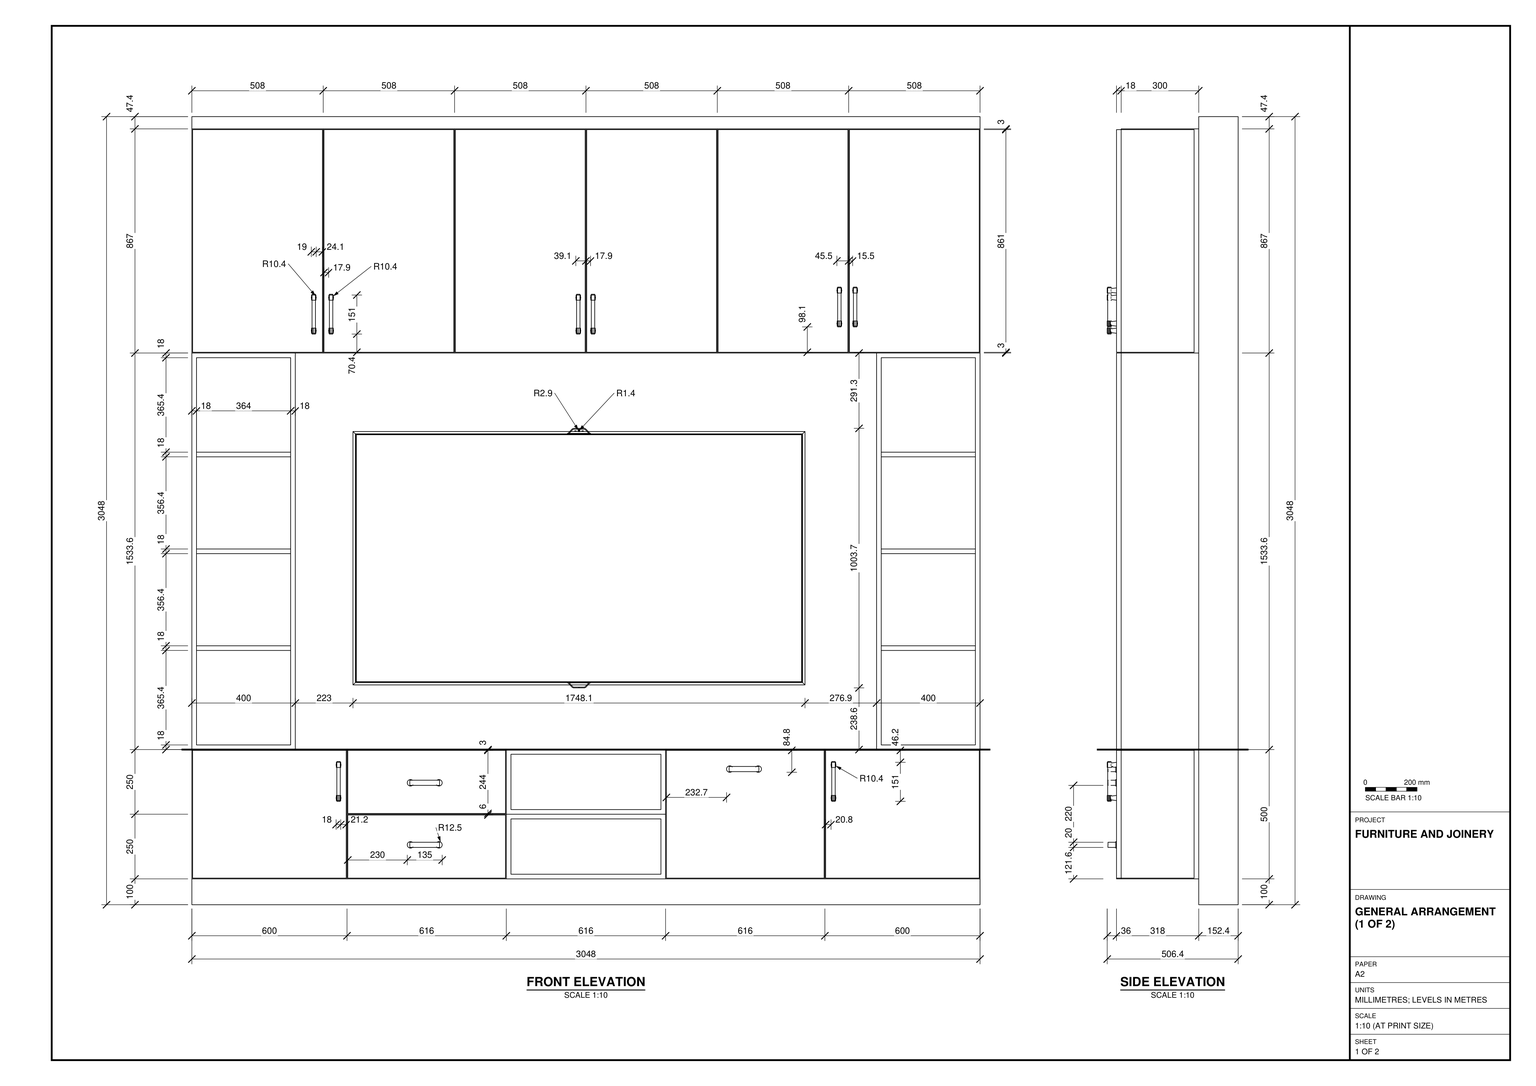
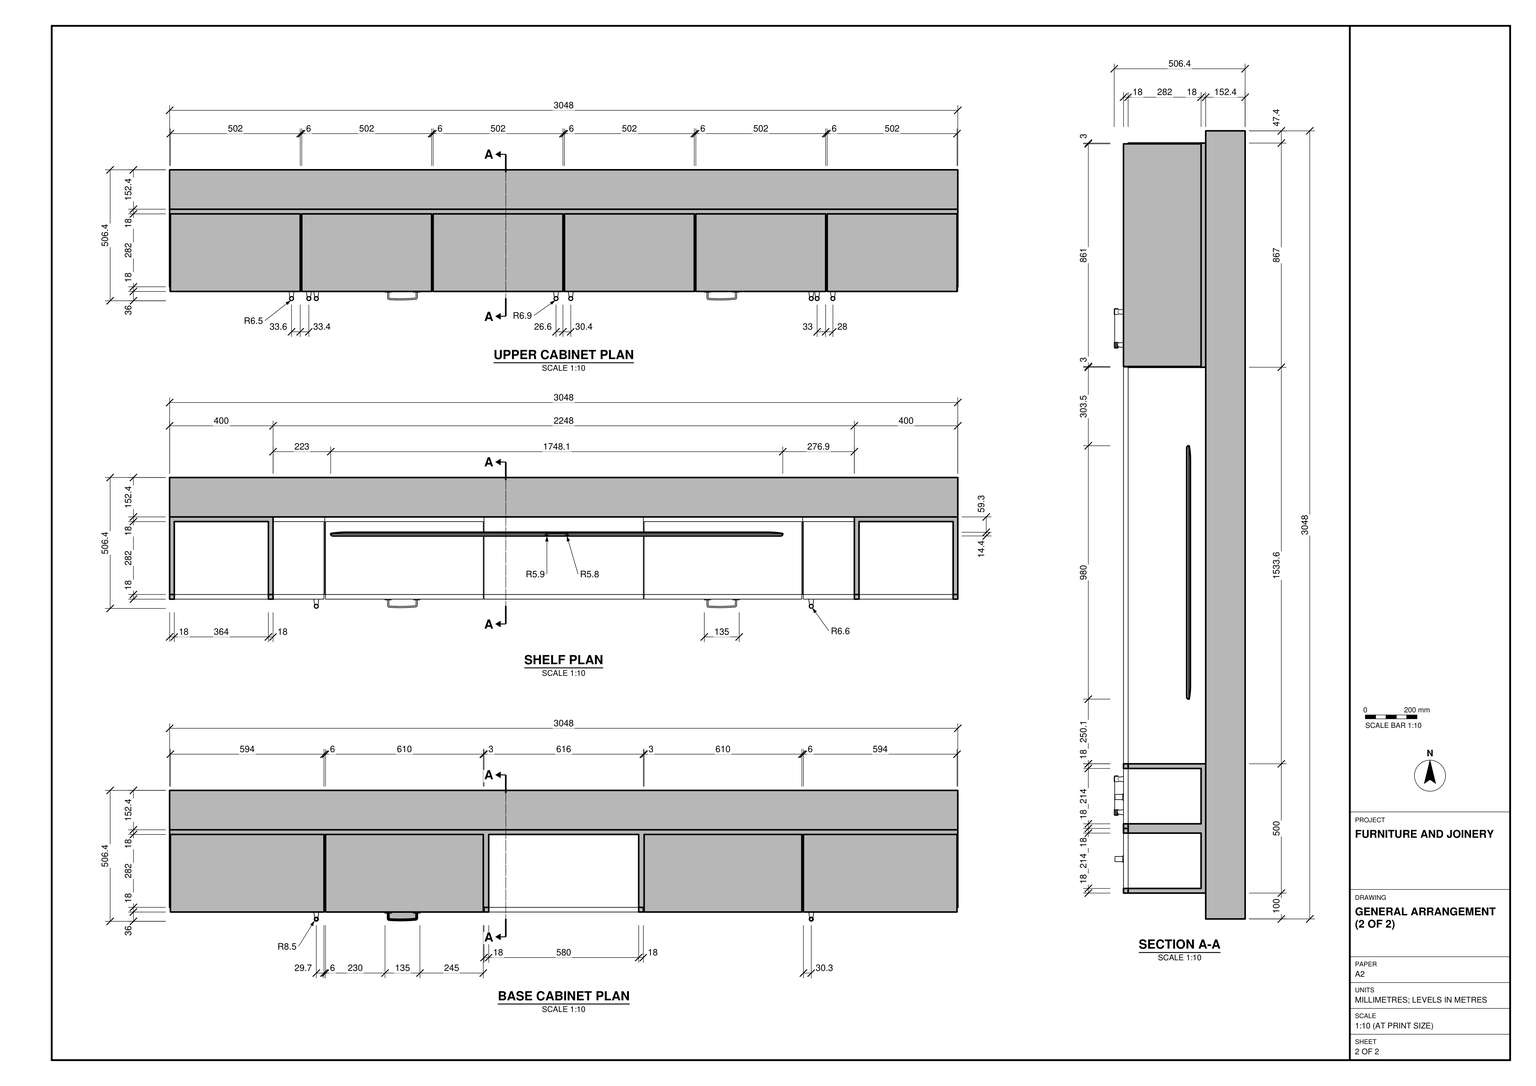
Build the television wall unit in SketchUp from task_files/diagram_01.pdf. Work in millimetres and use 0 mm as the floor datum. The complete assembly is 3048 mm wide, 506.4 mm deep and 3048 mm high. Use the front elevation to lay out the cabinet fronts and the plans and section to set their depths relative to the 152.4 mm thick backing wall.

Set the base cabinets 100 mm above the floor. Across the base, model an end cupboard, two stacked drawers, two stacked open compartments, a single full-height front and the other end cupboard, in that order. Above the base, build a 400 mm wide open shelving tower at each end. Mount the television against the backing between the towers, leaving the slightly larger clearance on its right shown in the shelf plan. Span the full width above the towers with six upper cabinet doors. Match the panel thicknesses, gaps between fronts and handle positions to the drawings.

Keep the backing wall, cabinet assemblies, shelving towers and television as separate groups or components, and use components for repeated parts such as shelves and handles. Decor and loose items, including the television, may use any suitable library component. Save one SketchUp model as output_files/television_wall_unit_with_cabinets_and_open_shelving.skp.

# SketchUp Ruby script. Lengths in millimetres.
U = 1.mm
M = Sketchup.active_model
def pt(a) = Geom::Point3d.new(a.map { |v| v * U })
def face(e, loops, mat)
  f = e.add_face(loops[0].map { |a| pt(a) })
  loops[1..].each { |l| e.add_face(l.map { |a| pt(a) }).erase! }
  f.material = f.back_material = mat if mat
  f
end
# faces: each face lists its corners as indices into pts; further lists are holes
def faces(e, pts, list, mat = nil) = list.each { |f| face(e, (f[0].is_a?(Array) ? f : [f]).map { |l| l.map { |i| pts[i] } }, mat) }
# xy, xz, yz: faces in a plane at the given z, y or x. An outline is a flat list of corners, or four numbers for a rectangle; further outlines are holes
def ring(l) = l.size == 4 ? [[l[0], l[1]], [l[2], l[1]], [l[2], l[3]], [l[0], l[3]]] : l.each_slice(2).to_a
def flat(e, list, mat, &to3) = list.each { |f| face(e, (f[0].is_a?(Array) ? f : [f]).map { |l| ring(l).map { |u, v| to3.(u, v) } }, mat) }
def xy(e, z, list, mat = nil) = flat(e, list, mat) { |x, y| [x, y, z] }
def xz(e, y, list, mat = nil) = flat(e, list, mat) { |x, z| [x, y, z] }
def yz(e, x, list, mat = nil) = flat(e, list, mat) { |y, z| [x, y, z] }
def lines(e, pts, list) = list.each { |a, b| e.add_line(pt(pts[a]), pt(pts[b])) }
# prism: a flat outline (further loops are holes) pulled along v
def prism(e, loops, v, mat = nil)
  f = face(e, loops, mat); d = Geom::Vector3d.new(v.map { |x| x * U })
  f.pushpull(f.normal.samedirection?(d) ? d.length : -d.length)
end
def box(e, o, s, mat = nil) = prism(e, [[o, [o[0] + s[0], o[1], o[2]], [o[0] + s[0], o[1] + s[1], o[2]], [o[0], o[1] + s[1], o[2]]]], [0, 0, s[2]], mat)
def at(x, y, z, deg = 0) = Geom::Transformation.translation(pt([x, y, z])) * Geom::Transformation.rotation(ORIGIN, Z_AXIS, deg.degrees)
def axes(o, x, y, z) = Geom::Transformation.new([*x, 0, *y, 0, *z, 0, *pt(o).to_a, 1])
def part(name) = M.definitions.add(name)
# library, detail: a bought-in or finely detailed component or shape, given as its bounding box
def library(name, o, s) = part(name).tap { |d| box(d.entities, o, s) }
def detail(e, o, s) = box(e.add_group.entities, o, s)
def put(e, d, t, mat = nil) = e.add_instance(d, t).tap { |i| i.material = mat if mat }
def group(e, t, mat = nil) = e.add_group.tap { |g| g.transformation = t; g.material = mat if mat }.entities
root = M.entities
M.materials.add("[0137_Black]").color = [0, 0, 0]
c1 = library("download?mid=50c7180b9fccec56d493bfe20f94b6ab&ctyp=sp&cv=p8.",[3795.5,1113.3,453.6],[1898.6,14.5,1067.8])
c2 = library("1-POIGNEE CLC2",[-77,-9.5,0],[154,19,36])
c3 = library("2-POIGNEE CLC2",[-67.5,-12.5,0],[135,25,33])
put(root,c1,axes([-2871.5,-869.1,412.2],[0.9207,0,0],[0,1,0],[0,0,0.94]))
put(root,c2,axes([471.4,0,2284],[0,0,1],[-1,0,0],[0,-1,0]))
put(root,c2,axes([538.4,0,2284],[0,0,1],[-1,0,0],[0,-1,0]))
put(root,c2,axes([1494.4,0,2284],[0,0,1],[-1,0,0],[0,-1,0]))
put(root,c2,axes([1551.4,0,2284],[0,0,1],[-1,0,0],[0,-1,0]))
put(root,c2,axes([2504,0,2311.7],[0,0,1],[-1,0,0],[0,-1,0]))
put(root,c2,axes([2565,0,2311.7],[0,0,1],[-1,0,0],[0,-1,0]))
put(root,c2,axes([567.3,0,476.8],[0,0,1],[-1,0,0],[0,-1,0]))
put(root,c3,axes([900.5,0,471.6],[1,0,0],[0,0,1],[0,-1,0]))
put(root,c3,axes([900.5,0,231.6],[1,0,0],[0,0,1],[0,-1,0]))
put(root,c2,axes([2481.3,0,476.8],[0,0,1],[-1,0,0],[0,-1,0]))
put(root,c3,axes([2135.2,0,524.7],[1,0,0],[0,0,1],[0,-1,0]))
g1 = group(root,at(0,318,0))
box(g1,[0,0,0],[3048,152.4,3048])
g2 = group(root,at(0,18,100))
xy(g2,0,[[1216,-18,1832,0],[0,0,3048,300]])
xy(g2,3,[[3,0,597,282],[603,0,1213,282],[1835,0,2445,282],[2451,0,3045,282]])
xy(g2,18,[[1234,-18,1814,0],[1234,0,1814,282]])
xy(g2,232,[[1234,-18,1814,0],[1234,0,1814,282]])
xy(g2,247,[[603,0,1213,282]])
xy(g2,250,[[1216,-18,1832,0]])
xy(g2,253,[[603,0,1213,282]])
xy(g2,268,[[1234,-18,1814,0],[1234,0,1814,282]])
xy(g2,482,[[1234,-18,1814,0],[1234,0,1814,282]])
xy(g2,497,[[3,0,597,282],[603,0,1213,282],[1835,0,2445,282],[2451,0,3045,282]])
xy(g2,500,[[1216,-18,1832,0],[0,0,600,300],[600,0,1216,300],[1216,0,1832,300],[1832,0,2448,300],
  [2448,0,3048,300]])
xz(g2,-18,[[[1216,0,1832,250],[1234,18,1814,232]],[[1216,250,1832,500],[1234,268,1814,482]]],"[0137_Black]")
xz(g2,0,[[[0,0,600,500],[3,3,597,497]],[[600,0,1216,250],[603,3,1213,247]],[[1216,0,1832,250],[1234,18,1814,232]],[[1832,0,2448,500],[1835,3,2445,497]],[[2448,0,3048,500],[2451,3,3045,497]],
  [[600,250,1216,500],[603,253,1213,497]],[[1216,250,1832,500],[1234,268,1814,482]]])
xz(g2,282,[[3,3,597,497],[603,3,1213,247],[1835,3,2445,497],[2451,3,3045,497],[1234,18,1814,232],
  [603,253,1213,497],[1234,268,1814,482]])
xz(g2,300,[[0,0,3048,500]])
yz(g2,0,[[0,0,300,500]])
yz(g2,3,[[0,3,282,497]])
yz(g2,597,[[0,3,282,497]])
yz(g2,603,[[0,3,282,247],[0,253,282,497]])
yz(g2,1213,[[0,3,282,247],[0,253,282,497]])
yz(g2,1216,[[-18,0,0,250],[-18,250,0,500]])
yz(g2,1234,[[-18,18,0,232],[0,18,282,232],[-18,268,0,482],[0,268,282,482]])
yz(g2,1814,[[-18,18,0,232],[0,18,282,232],[-18,268,0,482],[0,268,282,482]])
yz(g2,1832,[[-18,0,0,250],[-18,250,0,500]])
yz(g2,1835,[[0,3,282,250],[0,250,282,497]])
yz(g2,2445,[[0,3,282,497]])
yz(g2,2451,[[0,3,282,497]])
yz(g2,3045,[[0,3,282,497]])
yz(g2,3048,[[0,0,300,500]])
g3 = group(root,at(0,0,100))
xy(g3,3,[[3,0,597,18]])
xy(g3,497,[[3,0,597,18]])
xz(g3,0,[[3,3,597,497]])
xz(g3,18,[[[0,0,600,500],[3,3,597,497]]])
yz(g3,3,[[0,3,18,497]])
yz(g3,597,[[0,3,18,497]])
g4 = group(root,at(600,0,350))
xy(g4,3,[[3,0,613,18]])
xy(g4,247,[[3,0,613,18]])
xz(g4,0,[[3,3,613,247]])
xz(g4,18,[[[0,0,616,250],[3,3,613,247]]])
yz(g4,3,[[0,3,18,247]])
yz(g4,613,[[0,3,18,247]])
g5 = group(root,at(600,0,100))
xy(g5,3,[[3,0,613,18]])
xy(g5,247,[[3,0,613,18]])
xz(g5,0,[[3,3,613,247]])
xz(g5,18,[[[0,0,616,250],[3,3,613,247]]])
yz(g5,3,[[0,3,18,247]])
yz(g5,613,[[0,3,18,247]])
g6 = group(root,at(1832,0,100))
xy(g6,3,[[3,0,613,18]])
xy(g6,497,[[3,0,613,18]])
xz(g6,0,[[3,3,613,497]])
xz(g6,18,[[[0,0,616,500],[3,3,613,497]]])
yz(g6,3,[[0,3,18,497]])
yz(g6,613,[[0,3,18,497]])
g7 = group(root,at(2448,0,100))
xy(g7,3,[[3,0,597,18]])
xy(g7,497,[[3,0,597,18]])
xz(g7,0,[[3,3,597,497]])
xz(g7,18,[[[0,0,600,500],[3,3,597,497]]])
yz(g7,3,[[0,3,18,497]])
yz(g7,597,[[0,3,18,497]])
g8 = group(root,at(0,18,600))
xy(g8,0,[[0,-18,400,0],[0,0,400,300]])
xy(g8,18,[[18,-18,382,0],[18,0,382,282]])
xy(g8,383.4,[[18,0,382,282]])
xy(g8,401.4,[[18,0,382,282]])
xy(g8,757.8,[[18,0,382,282]])
xy(g8,775.8,[[18,0,382,282]])
xy(g8,1132.2,[[18,0,382,282]])
xy(g8,1150.2,[[18,0,382,282]])
xy(g8,1515.6,[[18,-18,382,0],[18,0,382,282]])
xy(g8,1533.6,[[0,-18,400,0],[0,0,400,300]])
xz(g8,-18,[[[0,0,400,1533.6],[18,18,382,1515.6]]])
xz(g8,0,[[[0,0,400,1533.6],[18,18,382,1515.6]],[18,383.4,382,401.4],[18,757.8,382,775.8],[18,1132.2,382,1150.2]])
xz(g8,282,[[18,18,382,383.4],[18,401.4,382,757.8],[18,775.8,382,1132.2],[18,1150.2,382,1515.6]])
xz(g8,300,[[0,0,400,1533.6]])
yz(g8,0,[[-18,0,0,1533.6],[0,0,300,1533.6]])
yz(g8,18,[[-18,18,0,1515.6],[0,18,282,383.4],[0,401.4,282,757.8],[0,775.8,282,1132.2],[0,1150.2,282,1515.6]])
yz(g8,382,[[-18,18,0,1515.6],[0,18,282,383.4],[0,401.4,282,757.8],[0,775.8,282,1132.2],[0,1150.2,282,1515.6]])
yz(g8,400,[[-18,0,0,1533.6],[0,0,300,1533.6]])
g9 = group(root,at(2648,18,600))
xy(g9,0,[[0,-18,400,0],[0,0,400,300]])
xy(g9,18,[[18,-18,382,0],[18,0,382,282]])
xy(g9,383.4,[[18,0,382,282]])
xy(g9,401.4,[[18,0,382,282]])
xy(g9,757.8,[[18,0,382,282]])
xy(g9,775.8,[[18,0,382,282]])
xy(g9,1132.2,[[18,0,382,282]])
xy(g9,1150.2,[[18,0,382,282]])
xy(g9,1515.6,[[18,-18,382,0],[18,0,382,282]])
xy(g9,1533.6,[[0,-18,400,0],[0,0,400,300]])
xz(g9,-18,[[[0,0,400,1533.6],[18,18,382,1515.6]]])
xz(g9,0,[[[0,0,400,1533.6],[18,18,382,1515.6]],[18,383.4,382,401.4],[18,757.8,382,775.8],[18,1132.2,382,1150.2]])
xz(g9,282,[[18,18,382,383.4],[18,401.4,382,757.8],[18,775.8,382,1132.2],[18,1150.2,382,1515.6]])
xz(g9,300,[[0,0,400,1533.6]])
yz(g9,0,[[-18,0,0,1533.6],[0,0,300,1533.6]])
yz(g9,18,[[-18,18,0,1515.6],[0,18,282,383.4],[0,401.4,282,757.8],[0,775.8,282,1132.2],[0,1150.2,282,1515.6]])
yz(g9,382,[[-18,18,0,1515.6],[0,18,282,383.4],[0,401.4,282,757.8],[0,775.8,282,1132.2],[0,1150.2,282,1515.6]])
yz(g9,400,[[-18,0,0,1533.6],[0,0,300,1533.6]])
g10 = group(root,at(0,18,2133.6))
xy(g10,0,[[0,0,3048,300]])
xy(g10,3,[[3,0,505,282],[511,0,1013,282],[1019,0,1521,282],[1527,0,2029,282],[2035,0,2537,282],
  [2543,0,3045,282]])
xy(g10,864,[[3,0,505,282],[511,0,1013,282],[1019,0,1521,282],[1527,0,2029,282],[2035,0,2537,282],
  [2543,0,3045,282]])
xy(g10,867,[[0,0,3048,300]])
xz(g10,0,[[[0,0,508,867],[3,3,505,864]],[[508,0,1016,867],[511,3,1013,864]],[[1016,0,1524,867],[1019,3,1521,864]],[[1524,0,2032,867],[1527,3,2029,864]],[[2032,0,2540,867],[2035,3,2537,864]],
  [[2540,0,3048,867],[2543,3,3045,864]]])
xz(g10,282,[[3,3,505,864],[511,3,1013,864],[1019,3,1521,864],[1527,3,2029,864],[2035,3,2537,864],
  [2543,3,3045,864]])
xz(g10,300,[[0,0,3048,867]])
yz(g10,0,[[0,0,300,867]])
yz(g10,3,[[0,3,282,864]])
yz(g10,505,[[0,3,282,864]])
yz(g10,511,[[0,3,282,864]])
yz(g10,1013,[[0,3,282,864]])
yz(g10,1019,[[0,3,282,864]])
yz(g10,1521,[[0,3,282,864]])
yz(g10,1527,[[0,3,282,864]])
yz(g10,2029,[[0,3,282,864]])
yz(g10,2035,[[0,3,282,864]])
yz(g10,2537,[[0,3,282,864]])
yz(g10,2543,[[0,3,282,864]])
yz(g10,3045,[[0,3,282,864]])
yz(g10,3048,[[0,0,300,867]])
g11 = group(root,at(0,0,2133.6))
xy(g11,3,[[3,0,505,18]])
xy(g11,864,[[3,0,505,18]])
xz(g11,0,[[3,3,505,864]])
xz(g11,18,[[[0,0,508,867],[3,3,505,864]]])
yz(g11,3,[[0,3,18,864]])
yz(g11,505,[[0,3,18,864]])
g12 = group(root,at(508,0,2133.6))
xy(g12,3,[[3,0,505,18]])
xy(g12,864,[[3,0,505,18]])
xz(g12,0,[[3,3,505,864]])
xz(g12,18,[[[0,0,508,867],[3,3,505,864]]])
yz(g12,3,[[0,3,18,864]])
yz(g12,505,[[0,3,18,864]])
g13 = group(root,at(1016,18,2133.6))
xy(g13,3,[[3,-18,505,0]])
xy(g13,864,[[3,-18,505,0]])
xz(g13,-18,[[3,3,505,864]])
xz(g13,0,[[[0,0,508,867],[3,3,505,864]]])
yz(g13,3,[[-18,3,0,864]])
yz(g13,505,[[-18,3,0,864]])
g14 = group(root,at(1524,0,2133.6))
xy(g14,3,[[3,0,505,18]])
xy(g14,864,[[3,0,505,18]])
xz(g14,0,[[3,3,505,864]])
xz(g14,18,[[[0,0,508,867],[3,3,505,864]]])
yz(g14,3,[[0,3,18,864]])
yz(g14,505,[[0,3,18,864]])
g15 = group(root,at(2032,0,2133.6))
xy(g15,3,[[3,0,505,18]])
xy(g15,864,[[3,0,505,18]])
xz(g15,0,[[3,3,505,864]])
xz(g15,18,[[[0,0,508,867],[3,3,505,864]]])
yz(g15,3,[[0,3,18,864]])
yz(g15,505,[[0,3,18,864]])
g16 = group(root,at(2540,0,2133.6))
xy(g16,3,[[3,0,505,18]])
xy(g16,864,[[3,0,505,18]])
xz(g16,0,[[3,3,505,864]])
xz(g16,18,[[[0,0,508,867],[3,3,505,864]]])
yz(g16,3,[[0,3,18,864]])
yz(g16,505,[[0,3,18,864]])
